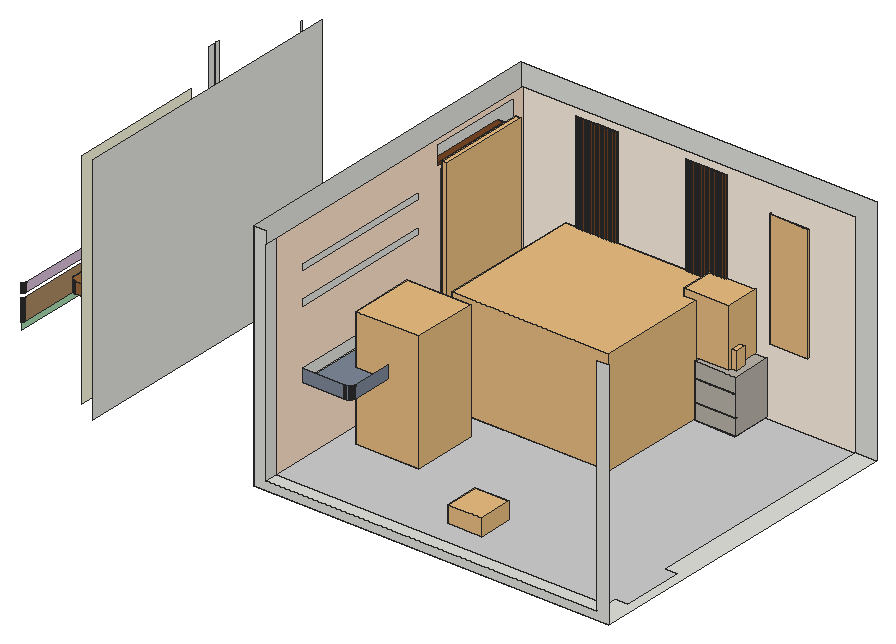
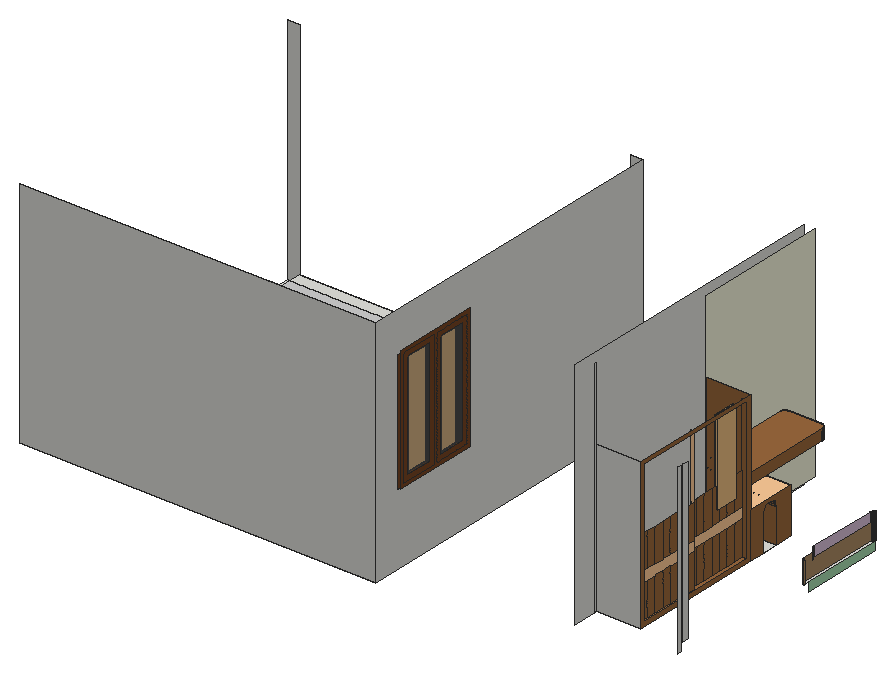
# SketchUp Ruby script. Lengths in inches.
U = 1.inch
M = Sketchup.active_model
def pt(a) = Geom::Point3d.new(a.map { |v| v * U })
def face(e, loops, mat)
  f = e.add_face(loops[0].map { |a| pt(a) })
  loops[1..].each { |l| e.add_face(l.map { |a| pt(a) }).erase! }
  f.material = f.back_material = mat if mat
  f
end
# faces: each face lists its corners as indices into pts; further lists are holes
def faces(e, pts, list, mat = nil) = list.each { |f| face(e, (f[0].is_a?(Array) ? f : [f]).map { |l| l.map { |i| pts[i] } }, mat) }
# xy, xz, yz: faces in a plane at the given z, y or x. An outline is a flat list of corners, or four numbers for a rectangle; further outlines are holes
def ring(l) = l.size == 4 ? [[l[0], l[1]], [l[2], l[1]], [l[2], l[3]], [l[0], l[3]]] : l.each_slice(2).to_a
def flat(e, list, mat, &to3) = list.each { |f| face(e, (f[0].is_a?(Array) ? f : [f]).map { |l| ring(l).map { |u, v| to3.(u, v) } }, mat) }
def xy(e, z, list, mat = nil) = flat(e, list, mat) { |x, y| [x, y, z] }
def xz(e, y, list, mat = nil) = flat(e, list, mat) { |x, z| [x, y, z] }
def yz(e, x, list, mat = nil) = flat(e, list, mat) { |y, z| [x, y, z] }
def lines(e, pts, list) = list.each { |a, b| e.add_line(pt(pts[a]), pt(pts[b])) }
# prism: a flat outline (further loops are holes) pulled along v
def prism(e, loops, v, mat = nil)
  f = face(e, loops, mat); d = Geom::Vector3d.new(v.map { |x| x * U })
  f.pushpull(f.normal.samedirection?(d) ? d.length : -d.length)
end
def box(e, o, s, mat = nil) = prism(e, [[o, [o[0] + s[0], o[1], o[2]], [o[0] + s[0], o[1] + s[1], o[2]], [o[0], o[1] + s[1], o[2]]]], [0, 0, s[2]], mat)
def at(x, y, z, deg = 0) = Geom::Transformation.translation(pt([x, y, z])) * Geom::Transformation.rotation(ORIGIN, Z_AXIS, deg.degrees)
def axes(o, x, y, z) = Geom::Transformation.new([*x, 0, *y, 0, *z, 0, *pt(o).to_a, 1])
def part(name) = M.definitions.add(name)
# library, detail: a bought-in or finely detailed component or shape, given as its bounding box
def library(name, o, s) = part(name).tap { |d| box(d.entities, o, s) }
def detail(e, o, s) = box(e.add_group.entities, o, s)
def put(e, d, t, mat = nil) = e.add_instance(d, t).tap { |i| i.material = mat if mat }
def group(e, t, mat = nil) = e.add_group.tap { |g| g.transformation = t; g.material = mat if mat }.entities
root = M.entities
M.materials.add("Leather K01 Brown 12cm").color = [167, 219, 175]
M.materials.add("Maquette Wood B01 12cm\#2").color = [172, 139, 100]
M.materials.add("Stone E 150cm").color = [186, 180, 170]
M.materials.add("[0049_Beige]").color = [245, 245, 220]
M.materials.add("[0090_LightCyan]").color = [224, 255, 255]
M.materials.add("[0110_LightSlateGray]").color = [127, 136, 153]
M.materials.add("[0110_LightSlateGray]1").color = [119, 136, 153]
M.materials.add("[0118_Thistle]").color = [216, 191, 216]
M.materials.add("[Carrera Marble]1").color = [207, 207, 207]
M.materials.add("[Color C01]").color = [255, 229, 204]
M.materials.add("[Color C02]").color = [255, 204, 153]
M.materials.add("[Color D01]").color = [255, 242, 228]
M.materials.add("[Translucent Glass Gray]").color = [132, 132, 132]
M.materials["[Translucent Glass Gray]"].alpha = 0.25
M.materials.add("[Wood Floor]").color = [155, 105, 61]
M.materials.add("[Wood Veneer 01]").color = [120, 70, 37]
c1 = library("Group\#3",[-0.5,-0.5,0],[2.0625,15.625,59.375])
c2 = part("Group\#33")
xy(c2.entities,0,[[0,0,19.69,1.18]],"[Wood Veneer 01]")
xy(c2.entities,2.76,[[2.76,0,16.93,1.18]],"[Wood Veneer 01]")
xy(c2.entities,60.24,[[2.76,0,16.93,1.18]],"[Wood Veneer 01]")
xy(c2.entities,62.99,[[0,0,19.69,1.18]],"[Wood Veneer 01]")
xz(c2.entities,0,[[2.76,2.76,16.93,60.24]],"[Translucent Glass Gray]")
xz(c2.entities,0,[[[0,0,19.69,62.99],[2.76,2.76,16.93,60.24]]],"[Wood Veneer 01]")
xz(c2.entities,1.18,[[[0,0,19.69,62.99],[2.76,2.76,16.93,60.24]]],"[Wood Veneer 01]")
yz(c2.entities,0,[[0,0,1.18,62.99]],"[Wood Veneer 01]")
yz(c2.entities,2.76,[[0,2.76,1.18,60.24]],"[Wood Veneer 01]")
yz(c2.entities,16.93,[[0,2.76,1.18,60.24]],"[Wood Veneer 01]")
yz(c2.entities,19.69,[[0,0,1.18,62.99]],"[Wood Veneer 01]")
c3 = part("pintu 2")
put(c3.entities,c2,at(-21.65,-1.97,1.97,-90))
g1 = group(c3.entities,at(-21.65,0,0,-90))
prism(g1,[[[0,0,66.93],[0,0,0],[45.28,0,0],[45.28,0,66.93]],[[43.31,0,1.97],[23.62,0,1.97],[23.62,0,64.96],[43.31,0,64.96]],[[21.65,0,64.96],[21.65,0,1.97],[1.97,0,1.97],[1.97,0,64.96]]],[0,5.91,0],"[Wood Veneer 01]")
put(c3.entities,c2,at(-21.65,-23.62,1.97,-90))
c4 = part("jendela")
put(c4.entities,c3,axes([-219.28,-83.75,50.21],[0.9198,0,0],[0,1.36117,0],[0,0,1.3104]))
c5 = library("Curtains\#1",[0,0,0],[121.73,8.19,117.22])
c6 = library("Chair 233 024",[-11.33,-15.06,-0.01],[22.66,30.64,41.53])
c7 = library("Bed 49-09",[-38.66,-44.09,0],[77.05,88.65,36.46])
c8 = library("Dome Light\#1",[-12,-12,0],[24,24,12])
c9 = library("Vase 004",[-7.23,-6.39,-0.02],[13.74,12.68,17.81])
c10 = library("Candle 296 009",[-1.31,-1.31,-0.01],[2.62,2.62,4.3])
c11 = library("Group\#8",[-0.5,-0.5,0],[27.375,1.5625,82.0625])
xy(root,0,[[314.72,0,566.72,236.75]])
xy(root,6.125,[[323.37,0,558.07,8.65],[467.82,201.17,495.07,228.1]])
xy(root,6.125,[[323.37,8.65,558.07,8.65,558.07,16.33,566.72,16.33,566.72,59.9,558.07,59.9,558.07,228.1,323.37,228.1]],"[Carrera Marble]1")
xy(root,7.125,[[467.07,200.35,467.82,228.1],[467.82,200.35,496.26,201.17],[495.07,201.17,496.26,228.1]])
xy(root,7.375,[[159.88,62.61,191.32,98.61]])
xy(root,10.06,[[159.88,101.5625,163.32,101.5625,163.32,147.01,161.57,147.01,161.57,192.875,159.88,192.875]],"[Wood Floor]")
xy(root,13.375,[[113.43,46.51,113.43,109,113.57,108.99,113.82,108.94,114.07,108.86,114.31,108.74,114.52,108.6,114.72,108.43,114.89,108.23,115.04,108.01,115.15,107.78,115.24,107.53,115.29,107.27,115.31,107.01,115.31,47.45,115.29,47.2,115.24,46.95,115.16,46.71,115.06,46.51],[113.43,109,113.43,109.01,113.31,109.01]])
xy(root,17.92,[[467.07,200.35,496.26,201.73]],"[0110_LightSlateGray]1")
xy(root,18.625,[[467.07,200.35,496.26,201.73]],"[0110_LightSlateGray]1")
xy(root,33.36,[[467.07,200.35,496.26,201.42]],"[0110_LightSlateGray]1")
xy(root,34.0625,[[467.07,200.35,496.26,201.42]],"[0110_LightSlateGray]1")
xy(root,44.375,[[467.07,200.35,496.26,228.1]],"Stone E 150cm")
xy(root,50.21,[[314.72,153.92,323.37,217.92]])
xy(root,54.08,[[360.9375,227.98,375.125,228.1],[439.0625,227.98,453.25,228.1]])
xy(root,54.08,[[376.0625,227.98,390.25,228.1],[453.8125,227.98,468,228.1]],"[0090_LightCyan]")
xy(root,54.9,[[323.37,31.6,323.37,123.51,353.74,123.51,354.39,123.47,355.03,123.36,355.65,123.17,356.24,122.92,356.78,122.6,357.28,122.22,357.71,121.79,358.07,121.31,358.36,120.79,358.57,120.25,358.7,119.68,358.74,119.11,358.74,36,358.7,35.43,358.57,34.86,358.36,34.32,358.07,33.8,357.71,33.33,357.28,32.89,356.78,32.51,356.24,32.19,355.65,31.9375,355.03,31.75,354.39,31.64,353.74,31.6]],"[0110_LightSlateGray]")
xy(root,54.9375,[[362.14,227.98,362.96,228.1]])
xy(root,54.9375,[[362.14,227.04,362.96,227.98],[364,227.04,364.83,228.1],[365.86,227.04,366.69,228.1],[367.73,227.04,368.55,228.1],[369.59,227.04,370.42,228.1],
  [371.46,227.04,372.28,228.1],[373.32,227.04,374.15,228.1],[377.14,227.04,377.96,228.1],[379,227.04,379.83,228.1],[380.86,227.04,381.69,228.1],
  [382.73,227.04,383.55,228.1],[384.59,227.04,385.42,228.1],[386.46,227.04,387.28,228.1],[388.32,227.04,389.15,228.1],[440.07,227.04,440.9,228.1],
  [441.9375,227.04,442.76,228.1],[443.8,227.04,444.63,228.1],[445.67,227.04,446.49,228.1],[447.53,227.04,448.36,228.1],[449.4,227.04,450.22,228.1],
  [451.26,227.04,452.09,228.1],[455.01,227.04,455.84,227.98],[456.88,227.04,457.71,228.1],[458.76,227.04,459.58,228.1],[460.63,227.04,461.45,228.1],
  [462.5,227.04,463.33,228.1],[464.375,227.04,465.2,228.1],[466.25,227.04,467.07,228.1],[455.01,227.98,455.84,228.1]],"[Wood Veneer 01]")
xy(root,55.6875,[[164.87,30.24,164.22,30.28,163.58,30.41,162.96,30.62,162.375,30.9,161.83,31.27,161.34,31.7,160.91,32.1875,160.55,32.73,160.26,33.3125,160.05,33.93,159.92,34.57,159.88,35.22,159.88,98.61,191.32,98.61,191.32,35.24,191.28,34.58,191.15,33.94,190.9375,33.32,190.65,32.74,190.29,32.19,189.86,31.7,189.36,31.27,188.82,30.91,188.23,30.62,187.61,30.41,186.97,30.28,186.32,30.24]],"[Wood Floor]")
xy(root,63.3125,[[164.87,30.24,186.32,30.24,186.97,30.28,187.61,30.41,188.23,30.62,188.82,30.91,189.36,31.27,189.86,31.7,190.29,32.19,190.65,32.74,190.9375,33.32,191.15,33.94,191.28,34.58,191.32,35.24,191.32,98.61,159.88,98.61,159.88,35.22,159.92,34.57,160.05,33.93,160.26,33.3125,160.55,32.73,160.91,32.1875,161.34,31.7,161.83,31.27,162.375,30.9,162.96,30.62,163.58,30.41,164.22,30.28]],"[Wood Floor]")
xy(root,150.4375,[[362.14,227.98,362.96,228.1]])
xy(root,150.4375,[[362.14,227.04,362.96,227.98],[364,227.04,364.83,228.1],[365.86,227.04,366.69,228.1],[367.73,227.04,368.55,228.1],[369.59,227.04,370.42,228.1],
  [371.46,227.04,372.28,228.1],[373.32,227.04,374.15,228.1],[377.14,227.04,377.96,228.1],[379,227.04,379.83,228.1],[380.86,227.04,381.69,228.1],
  [382.73,227.04,383.55,228.1],[384.59,227.04,385.42,228.1],[386.46,227.04,387.28,228.1],[388.32,227.04,389.15,228.1],[440.07,227.04,440.9,228.1],
  [441.9375,227.04,442.76,228.1],[443.8,227.04,444.63,228.1],[445.67,227.04,446.49,228.1],[447.53,227.04,448.36,228.1],[449.4,227.04,450.22,228.1],
  [451.26,227.04,452.09,228.1],[455.01,227.04,455.84,227.98],[456.88,227.04,457.71,228.1],[458.76,227.04,459.58,228.1],[460.63,227.04,461.45,228.1],
  [462.5,227.04,463.33,228.1],[464.375,227.04,465.2,228.1],[466.25,227.04,467.07,228.1],[455.01,227.98,455.84,228.1]],"[Wood Veneer 01]")
xy(root,150.83,[[360.9375,227.98,375.125,228.1],[376.0625,227.98,390.25,228.1],[439.0625,227.98,453.25,228.1],[453.8125,227.98,468,228.1]],"[0090_LightCyan]")
xz(root,0,[[314.72,0,566.72,0,566.72,164.75,558.07,164.75,558.07,6.125,323.37,6.125,323.37,164.75,314.72,164.75]])
xz(root,30.24,[[164.87,55.6875,186.32,63.3125]],"[Wood Floor]")
xz(root,31.6,[[323.37,54.9,353.74,63.71]],"[0110_LightSlateGray]")
xz(root,98.61,[[159.88,7.375,191.32,39.875],[159.88,55.6875,191.32,63.3125]])
xz(root,98.61,[[159.88,7.375,191.13,113.1875]],"[Wood Floor]")
xz(root,101.5625,[[159.88,10.06,163.32,110.51]],"[Wood Floor]")
xz(root,123.51,[[323.37,54.9,353.74,63.71]],"[0110_LightSlateGray]")
xz(root,147.01,[[161.57,10.06,163.32,110.51]],"[Color C02]")
xz(root,153.92,[[314.72,50.21,323.37,136.125]])
xz(root,192.875,[[159.88,10.06,161.57,110.51]],"[Wood Floor]")
xz(root,195.82,[[159.88,7.375,191.32,113.1875]])
xz(root,200.35,[[467.07,7.125,496.26,17.92],[467.07,18.625,496.26,33.36],[467.07,34.0625,496.26,44.375]],"Stone E 150cm")
xz(root,201.17,[[467.82,6.125,495.07,7.125]],"[0110_LightSlateGray]1")
xz(root,201.42,[[467.07,33.36,496.26,34.0625]],"[0110_LightSlateGray]1")
xz(root,201.73,[[467.07,17.92,496.26,18.625]],"[0110_LightSlateGray]1")
xz(root,217.92,[[314.72,50.21,323.37,136.125]])
xz(root,227.04,[[362.14,54.9375,362.96,150.4375],[364,54.9375,364.83,150.4375],[365.86,54.9375,366.69,150.4375],[367.73,54.9375,368.55,150.4375],[369.59,54.9375,370.42,150.4375],
  [371.46,54.9375,372.28,150.4375],[373.32,54.9375,374.15,150.4375],[377.14,54.9375,377.96,150.4375],[379,54.9375,379.83,150.4375],[380.86,54.9375,381.69,150.4375],
  [382.73,54.9375,383.55,150.4375],[384.59,54.9375,385.42,150.4375],[386.46,54.9375,387.28,150.4375],[388.32,54.9375,389.15,150.4375],[440.07,54.9375,440.9,150.4375],
  [441.9375,54.9375,442.76,150.4375],[443.8,54.9375,444.63,150.4375],[445.67,54.9375,446.49,150.4375],[447.53,54.9375,448.36,150.4375],[449.4,54.9375,450.22,150.4375],
  [451.26,54.9375,452.09,150.4375],[455.01,54.9375,455.84,150.4375],[456.88,54.9375,457.71,150.4375],[458.76,54.9375,459.58,150.4375],[460.63,54.9375,461.45,150.4375],
  [462.5,54.9375,463.33,150.4375],[464.375,54.9375,465.2,150.4375],[466.25,54.9375,467.07,150.4375]],"[Wood Veneer 01]")
xz(root,227.98,[[[360.9375,54.08,375.125,150.83],[362.14,54.9375,362.96,150.4375]],[[376.0625,54.08,390.25,150.83],[377.26,54.9375,378.09,150.4375]],[[439.0625,54.08,453.25,150.83],[440.26,54.9375,441.09,150.4375]],[[453.8125,54.08,468,150.83],[455.01,54.9375,455.84,150.4375]]],"[0090_LightCyan]")
xz(root,228.1,[[467.82,6.125,467.82,7.125,467.07,7.125,467.07,44.375,496.26,44.375,496.26,7.125,495.07,7.125,495.07,6.125],[[360.9375,54.08,375.125,150.83],[362.14,54.9375,362.96,150.4375]],[362.14,54.9375,362.96,150.4375]])
xz(root,228.1,[[323.37,6.125,558.07,155.75]],"[Color D01]")
xz(root,236.75,[[314.72,0,566.72,164.75]])
yz(root,112.06,[[52.76,28.5,101.76,35]],"[0118_Thistle]")
yz(root,113.43,[[46.51,7.375,105.14,13.375]],"Leather K01 Brown 12cm")
yz(root,115.31,[[47.45,13.375,107.01,28.5]],"Maquette Wood B01 12cm\#2")
yz(root,125.77,[[203.13,7.375,205.19,125.75],[197.07,13.0625,200.94,125.75]])
yz(root,159.88,[[[98.61,7.375,195.82,113.1875],[101.5625,10.06,192.875,110.51]],[35.22,55.6875,98.61,63.3125]],"[Wood Floor]")
yz(root,161.57,[[147.01,34.06,192.875,41.06]],"[Color C02]")
yz(root,161.57,[[147.01,10.06,153.82,34.06],[153.82,10.06,160.63,34.06],[160.63,10.06,167.44,34.06],[167.44,10.06,174.25,34.06],[174.25,10.06,181.0625,34.06],
  [181.0625,10.06,187.875,34.06],[187.875,10.06,192.875,34.06],[147.01,41.06,153.82,65.06],[153.82,41.06,160.63,65.06],[160.63,41.06,167.44,65.06],
  [167.44,41.06,174.25,65.06],[174.25,41.06,181.0625,65.06],[181.0625,41.06,187.875,65.06],[187.875,41.06,192.875,65.06]],"[Wood Floor]")
yz(root,163.32,[[101.5625,34.06,147.01,41.06]],"[Color C02]")
yz(root,163.32,[[101.5625,10.06,108.3,34.06],[108.3,10.06,115.04,34.06],[115.04,10.06,121.79,34.06],[121.79,10.06,128.53,34.06],[128.53,10.06,135.27,34.06],
  [135.27,10.06,142.01,34.06],[142.01,10.06,147.01,34.06],[101.5625,41.06,108.3,65.06],[108.3,41.06,108.3,65.06,109.82,65.06,109.82,57.32,110.31,55.66,111.16,54.15,112.35,52.88,113.79,51.93,115.04,51.47,115.04,41.06],[115.04,41.06,115.04,51.47,115.42,51.33,117.14,51.13,118.86,51.33,120.48,51.93,121.79,52.79,121.79,41.06],
  [121.79,41.06,121.79,52.79,121.93,52.88,123.11,54.15,123.96,55.66,124.45,57.32,124.45,65.06,128.53,65.06,128.53,41.06],[128.53,41.06,135.27,65.06],[135.27,41.06,142.01,65.06],[142.01,41.06,147.01,65.06]],"[Wood Floor]")
yz(root,191.13,[[2.25,7.375,98.61,164.75]],"[0049_Beige]")
yz(root,191.32,[[62.61,7.375,98.61,39.875],[195.82,7.375,197.07,164.75],[35.24,55.6875,98.61,63.3125]])
yz(root,198.9375,[[2.25,0,205.19,164.75]])
yz(root,314.72,[[[0,0,236.75,164.75],[153.92,50.21,217.92,136.125]]])
yz(root,323.37,[[0,6.125,8.65,155.75]])
yz(root,323.37,[[[8.65,6.125,228.1,155.75],[153.92,50.21,217.92,136.125],[152.04,138.75,219.6,152.6875],[31.6,54.9,123.51,63.71],[31.6,102.15,136.04,107.71],[31.6,124.78,136.04,129.78]]],"[Color C01]")
yz(root,358.74,[[36,54.9,119.11,63.71]],"[0110_LightSlateGray]")
yz(root,360.9375,[[227.98,54.08,228.1,150.83]])
yz(root,362.14,[[227.98,54.9375,228.1,150.4375]])
yz(root,362.14,[[227.04,54.9375,227.98,150.4375]],"[Wood Veneer 01]")
yz(root,362.96,[[227.98,54.9375,228.1,150.4375]])
yz(root,362.96,[[227.04,54.9375,227.98,150.4375]],"[Wood Veneer 01]")
yz(root,364,[[227.04,54.9375,228.1,150.4375]],"[Wood Veneer 01]")
yz(root,364.83,[[227.04,54.9375,228.1,150.4375]],"[Wood Veneer 01]")
yz(root,365.86,[[227.04,54.9375,228.1,150.4375]],"[Wood Veneer 01]")
yz(root,366.69,[[227.04,54.9375,228.1,150.4375]],"[Wood Veneer 01]")
yz(root,367.73,[[227.04,54.9375,228.1,150.4375]],"[Wood Veneer 01]")
yz(root,368.55,[[227.04,54.9375,228.1,150.4375]],"[Wood Veneer 01]")
yz(root,369.59,[[227.04,54.9375,228.1,150.4375]],"[Wood Veneer 01]")
yz(root,370.42,[[227.04,54.9375,228.1,150.4375]],"[Wood Veneer 01]")
yz(root,371.46,[[227.04,54.9375,228.1,150.4375]],"[Wood Veneer 01]")
yz(root,372.28,[[227.04,54.9375,228.1,150.4375]],"[Wood Veneer 01]")
yz(root,373.32,[[227.04,54.9375,228.1,150.4375]],"[Wood Veneer 01]")
yz(root,374.15,[[227.04,54.9375,228.1,150.4375]],"[Wood Veneer 01]")
yz(root,375.125,[[227.98,54.08,228.1,150.83]],"[0090_LightCyan]")
yz(root,376.0625,[[227.98,54.08,228.1,150.83]],"[0090_LightCyan]")
yz(root,377.14,[[227.04,54.9375,228.1,150.4375]],"[Wood Veneer 01]")
yz(root,377.96,[[227.04,54.9375,228.1,150.4375]],"[Wood Veneer 01]")
yz(root,379,[[227.04,54.9375,228.1,150.4375]],"[Wood Veneer 01]")
yz(root,379.83,[[227.04,54.9375,228.1,150.4375]],"[Wood Veneer 01]")
yz(root,380.86,[[227.04,54.9375,228.1,150.4375]],"[Wood Veneer 01]")
yz(root,381.69,[[227.04,54.9375,228.1,150.4375]],"[Wood Veneer 01]")
yz(root,382.73,[[227.04,54.9375,228.1,150.4375]],"[Wood Veneer 01]")
yz(root,383.55,[[227.04,54.9375,228.1,150.4375]],"[Wood Veneer 01]")
yz(root,384.59,[[227.04,54.9375,228.1,150.4375]],"[Wood Veneer 01]")
yz(root,385.42,[[227.04,54.9375,228.1,150.4375]],"[Wood Veneer 01]")
yz(root,386.46,[[227.04,54.9375,228.1,150.4375]],"[Wood Veneer 01]")
yz(root,387.28,[[227.04,54.9375,228.1,150.4375]],"[Wood Veneer 01]")
yz(root,388.32,[[227.04,54.9375,228.1,150.4375]],"[Wood Veneer 01]")
yz(root,389.15,[[227.04,54.9375,228.1,150.4375]],"[Wood Veneer 01]")
yz(root,390.25,[[227.98,54.08,228.1,150.83]],"[0090_LightCyan]")
yz(root,439.0625,[[227.98,54.08,228.1,150.83]],"[0090_LightCyan]")
yz(root,440.07,[[227.04,54.9375,228.1,150.4375]],"[Wood Veneer 01]")
yz(root,440.9,[[227.04,54.9375,228.1,150.4375]],"[Wood Veneer 01]")
yz(root,441.9375,[[227.04,54.9375,228.1,150.4375]],"[Wood Veneer 01]")
yz(root,442.76,[[227.04,54.9375,228.1,150.4375]],"[Wood Veneer 01]")
yz(root,443.8,[[227.04,54.9375,228.1,150.4375]],"[Wood Veneer 01]")
yz(root,444.63,[[227.04,54.9375,228.1,150.4375]],"[Wood Veneer 01]")
yz(root,445.67,[[227.04,54.9375,228.1,150.4375]],"[Wood Veneer 01]")
yz(root,446.49,[[227.04,54.9375,228.1,150.4375]],"[Wood Veneer 01]")
yz(root,447.53,[[227.04,54.9375,228.1,150.4375]],"[Wood Veneer 01]")
yz(root,448.36,[[227.04,54.9375,228.1,150.4375]],"[Wood Veneer 01]")
yz(root,449.4,[[227.04,54.9375,228.1,150.4375]],"[Wood Veneer 01]")
yz(root,450.22,[[227.04,54.9375,228.1,150.4375]],"[Wood Veneer 01]")
yz(root,451.26,[[227.04,54.9375,228.1,150.4375]],"[Wood Veneer 01]")
yz(root,452.09,[[227.04,54.9375,228.1,150.4375]],"[Wood Veneer 01]")
yz(root,453.25,[[227.98,54.08,228.1,150.83]],"[0090_LightCyan]")
yz(root,453.8125,[[227.98,54.08,228.1,150.83]],"[0090_LightCyan]")
yz(root,455.01,[[227.04,54.9375,227.98,150.4375],[227.98,54.9375,228.1,150.4375]],"[Wood Veneer 01]")
yz(root,455.84,[[227.04,54.9375,227.98,150.4375],[227.98,54.9375,228.1,150.4375]],"[Wood Veneer 01]")
yz(root,456.88,[[227.04,54.9375,228.1,150.4375]],"[Wood Veneer 01]")
yz(root,457.71,[[227.04,54.9375,228.1,150.4375]],"[Wood Veneer 01]")
yz(root,458.76,[[227.04,54.9375,228.1,150.4375]],"[Wood Veneer 01]")
yz(root,459.58,[[227.04,54.9375,228.1,150.4375]],"[Wood Veneer 01]")
yz(root,460.63,[[227.04,54.9375,228.1,150.4375]],"[Wood Veneer 01]")
yz(root,461.45,[[227.04,54.9375,228.1,150.4375]],"[Wood Veneer 01]")
yz(root,462.5,[[227.04,54.9375,228.1,150.4375]],"[Wood Veneer 01]")
yz(root,463.33,[[227.04,54.9375,228.1,150.4375]],"[Wood Veneer 01]")
yz(root,464.375,[[227.04,54.9375,228.1,150.4375]],"[Wood Veneer 01]")
yz(root,465.2,[[227.04,54.9375,228.1,150.4375]],"[Wood Veneer 01]")
yz(root,466.25,[[227.04,54.9375,228.1,150.4375]],"[Wood Veneer 01]")
yz(root,467.07,[[200.35,7.125,200.35,17.92,201.73,17.92,201.73,18.625,200.35,18.625,200.35,33.36,201.42,33.36,201.42,34.0625,200.35,34.0625,200.35,44.375,228.1,44.375,228.1,7.125]],"Stone E 150cm")
yz(root,467.07,[[227.04,54.9375,228.1,150.4375]],"[Wood Veneer 01]")
yz(root,467.82,[[201.17,6.125,228.1,7.125]],"[0110_LightSlateGray]1")
yz(root,468,[[227.98,54.08,228.1,150.83]],"[0090_LightCyan]")
yz(root,495.07,[[201.17,6.125,228.1,7.125]],"[0110_LightSlateGray]1")
yz(root,496.26,[[200.35,7.125,228.1,7.125,228.1,44.375,200.35,44.375,200.35,34.0625,201.42,34.0625,201.42,33.36,200.35,33.36,200.35,18.625,201.73,18.625,201.73,17.92,200.35,17.92]],"Stone E 150cm")
p = [[113.62,45.53,28.5],[113.37,45.51,28.5],[113.37,45.51,13.375],[113.62,45.53,13.375],[113.87,45.58,28.5],[113.87,45.58,13.375],
  [114.11,45.66,28.5],[114.11,45.66,13.375],[114.34,45.77,28.5],[114.34,45.77,13.375],[114.55,45.91,28.5],[114.55,45.91,13.375],
  [114.74,46.08,28.5],[114.74,46.08,13.375],[114.9,46.27,28.5],[114.9,46.27,13.375],[115.05,46.48,28.5],[115.05,46.48,13.375],
  [115.16,46.71,28.5],[115.06,46.51,13.375],[115.16,46.71,13.375],[115.24,46.95,28.5],[115.24,46.95,13.375],[115.29,47.2,28.5],
  [115.29,47.2,13.375],[115.31,47.45,28.5],[115.31,47.45,13.375],[115.29,107.27,28.5],[115.31,107.01,28.5],[115.31,107.01,13.375],
  [115.29,107.27,13.375],[115.24,107.53,28.5],[115.24,107.53,13.375],[115.15,107.78,28.5],[115.15,107.78,13.375],[115.04,108.01,28.5],
  [115.04,108.01,13.375],[114.89,108.23,28.5],[114.89,108.23,13.375],[114.72,108.43,28.5],[114.72,108.43,13.375],[114.52,108.6,28.5],
  [114.52,108.6,13.375],[114.31,108.74,28.5],[114.31,108.74,13.375],[114.07,108.86,28.5],[114.07,108.86,13.375],[113.57,108.99,28.5],
  [113.82,108.94,28.5],[113.82,108.94,13.375],[113.57,108.99,13.375],[113.31,109.01,28.5],[113.43,109,13.375],[113.31,109.01,13.375],
  [110.49,49.59,35],[110.06,49.3,35],[110.06,49.3,28.5],[110.49,49.59,28.5],[110.88,49.93,35],[110.88,49.93,28.5],
  [111.23,50.33,35],[111.23,50.33,28.5],[111.52,50.76,35],[111.52,50.76,28.5],[111.75,51.23,35],[111.75,51.23,28.5],
  [111.92,51.73,35],[111.92,51.73,28.5],[112.02,52.24,35],[112.02,52.24,28.5],[112.06,52.76,35],[112.06,52.76,28.5],
  [112.02,102.28,35],[112.06,101.76,35],[112.06,101.76,28.5],[112.02,102.28,28.5],[111.92,102.8,35],[111.92,102.8,28.5],
  [111.75,103.29,35],[111.75,103.29,28.5],[111.52,103.76,35],[111.52,103.76,28.5],[111.23,104.2,35],[111.23,104.2,28.5],
  [110.88,104.59,35],[110.88,104.59,28.5],[110.49,104.93,35],[110.49,104.93,28.5],[110.06,105.22,35],[110.06,105.22,28.5],
  [163.32,117.14,51.13],[163.32,115.42,51.33],[162.26,115.42,51.33],[162.26,117.14,51.13],[163.32,118.86,51.33],[162.26,118.86,51.33],
  [163.32,115.04,51.47],[162.26,115.04,51.47],[163.32,120.48,51.93],[162.26,120.48,51.93],[163.32,121.79,52.79],[162.26,121.79,52.79],
  [163.32,121.93,52.88],[162.26,121.93,52.88],[163.32,123.11,54.15],[162.26,123.11,54.15],[163.32,123.96,55.66],[162.26,123.96,55.66],
  [354.39,31.64,63.71],[353.74,31.6,63.71],[353.74,31.6,54.9],[354.39,31.64,54.9],[355.03,31.75,63.71],[355.03,31.75,54.9],
  [355.65,31.9375,63.71],[355.65,31.9375,54.9],[356.24,32.19,63.71],[356.24,32.19,54.9],[356.78,32.51,63.71],[356.78,32.51,54.9],
  [357.28,32.89,63.71],[357.28,32.89,54.9],[357.71,33.33,63.71],[357.71,33.33,54.9],[358.07,33.8,63.71],[358.07,33.8,54.9],
  [358.36,34.32,63.71],[358.36,34.32,54.9],[358.57,34.86,63.71],[358.57,34.86,54.9],[358.7,35.43,63.71],[358.7,35.43,54.9],
  [358.74,36,63.71],[358.74,36,54.9],[358.7,119.68,63.71],[358.74,119.11,63.71],[358.74,119.11,54.9],[358.7,119.68,54.9],
  [358.57,120.25,63.71],[358.57,120.25,54.9],[358.36,120.79,63.71],[358.36,120.79,54.9],[358.07,121.31,63.71],[358.07,121.31,54.9],
  [357.71,121.79,63.71],[357.71,121.79,54.9],[357.28,122.22,63.71],[357.28,122.22,54.9],[356.78,122.6,63.71],[356.78,122.6,54.9],
  [356.24,122.92,63.71],[356.24,122.92,54.9],[355.65,123.17,63.71],[355.65,123.17,54.9],[355.03,123.36,63.71],[355.03,123.36,54.9],
  [354.39,123.47,63.71],[354.39,123.47,54.9],[353.74,123.51,63.71],[353.74,123.51,54.9],[164.87,30.24,63.3125],[164.22,30.28,63.3125],
  [164.22,30.28,55.6875],[164.87,30.24,55.6875],[186.97,30.28,63.3125],[186.32,30.24,63.3125],[186.32,30.24,55.6875],[186.97,30.28,55.6875],
  [163.58,30.41,63.3125],[163.58,30.41,55.6875],[187.61,30.41,63.3125],[187.61,30.41,55.6875],[162.96,30.62,63.3125],[162.96,30.62,55.6875],
  [188.23,30.62,63.3125],[188.23,30.62,55.6875],[162.375,30.9,63.3125],[162.375,30.9,55.6875],[188.82,30.91,63.3125],[188.82,30.91,55.6875],
  [161.83,31.27,63.3125],[161.83,31.27,55.6875],[189.36,31.27,63.3125],[189.36,31.27,55.6875],[161.34,31.7,63.3125],[161.34,31.7,55.6875],
  [189.86,31.7,63.3125],[189.86,31.7,55.6875],[160.91,32.1875,63.3125],[160.91,32.1875,55.6875],[190.29,32.19,63.3125],[190.29,32.19,55.6875],
  [160.55,32.73,63.3125],[160.55,32.73,55.6875],[190.65,32.74,63.3125],[190.65,32.74,55.6875],[160.26,33.3125,63.3125],[160.26,33.3125,55.6875],
  [190.9375,33.32,63.3125],[190.9375,33.32,55.6875],[160.05,33.93,63.3125],[160.05,33.93,55.6875],[191.15,33.94,63.3125],[191.15,33.94,55.6875],
  [159.92,34.57,63.3125],[159.92,34.57,55.6875],[191.28,34.58,63.3125],[191.28,34.58,55.6875],[159.88,35.22,63.3125],[159.88,35.22,55.6875],
  [191.32,35.24,63.3125],[191.32,35.24,55.6875],[163.32,124.45,57.32],[162.26,124.45,57.32]]
faces(root,p,[[0,1,2,3],[4,0,3,5],[6,4,5,7],[8,6,7,9],[10,8,9,11],[12,10,11,13],[14,12,13,15],[16,14,15,17],
  [18,16,17,19,20],[21,18,20,22],[23,21,22,24],[25,23,24,26],[27,28,29,30],[31,27,30,32],[33,31,32,34],[35,33,34,36],
  [37,35,36,38],[39,37,38,40],[41,39,40,42],[43,41,42,44],[45,43,44,46],[47,48,49,50],[48,45,46,49],[51,47,50,52,53]],"Maquette Wood B01 12cm\#2")
faces(root,p,[[54,55,56,57],[58,54,57,59],[60,58,59,61],[62,60,61,63],[64,62,63,65],[66,64,65,67],[68,66,67,69],[70,68,69,71]],"[0118_Thistle]")
faces(root,p,[[72,73,74,75],[76,72,75,77],[78,76,77,79],[80,78,79,81],[82,80,81,83],[84,82,83,85],[86,84,85,87],[88,86,87,89],
  [90,91,92,93],[94,90,93,95],[91,96,97,92],[98,94,95,99],[100,98,99,101],[102,100,101,103],[104,102,103,105],[106,104,105,107],
  [212,106,107,213]])
faces(root,p,[[108,109,110,111],[112,108,111,113],[114,112,113,115],[116,114,115,117],[118,116,117,119],[120,118,119,121],[122,120,121,123],[124,122,123,125],
  [126,124,125,127],[128,126,127,129],[130,128,129,131],[132,130,131,133],[134,135,136,137],[138,134,137,139],[140,138,139,141],[142,140,141,143],
  [144,142,143,145],[146,144,145,147],[148,146,147,149],[150,148,149,151],[152,150,151,153],[154,152,153,155],[156,154,155,157],[158,156,157,159]],"[0110_LightSlateGray]")
faces(root,p,[[160,161,162,163],[164,165,166,167],[161,168,169,162],[170,164,167,171],[168,172,173,169],[174,170,171,175],[172,176,177,173],[178,174,175,179],
  [176,180,181,177],[182,178,179,183],[180,184,185,181],[186,182,183,187],[184,188,189,185],[190,186,187,191],[188,192,193,189],[194,190,191,195],
  [192,196,197,193],[198,194,195,199],[196,200,201,197],[202,198,199,203],[200,204,205,201],[206,202,203,207],[204,208,209,205],[210,206,207,211]],"[Wood Floor]")
put(root,c1,at(162.26,109.82,51.13))
g2 = group(root,at(159.88,62.61,7.375))
xy(g2,0,[[0,12.8125,14,24.9375]],"[Wood Floor]")
xy(g2,32.5,[[0,0,31.4375,36]],"[Color C02]")
xz(g2,0,[[0,0,31.4375,32.5]],"[Wood Floor]")
xz(g2,12.8125,[[0,0,14,24.33]],"[Wood Floor]")
xz(g2,24.9375,[[0,0,14,24.33]],"[Wood Floor]")
yz(g2,0,[[0,0,0,32.5,36,32.5,36,0,24.9375,0,24.9375,24.33,24.73,25.9,24.125,27.36,23.16,28.62,21.91,29.58,20.44,30.1875,18.875,30.39,17.31,30.1875,15.84,29.58,14.59,28.62,13.625,27.36,13.02,25.9,12.8125,24.33,12.8125,0]],"[Wood Floor]")
yz(g2,14,[[12.8125,0,12.8125,24.33,13.02,25.9,13.625,27.36,14.59,28.62,15.84,29.58,17.31,30.1875,18.875,30.39,20.44,30.1875,21.91,29.58,23.16,28.62,24.125,27.36,24.73,25.9,24.9375,24.33,24.9375,0]],"[Wood Floor]")
p = [[0,12.8125,24.33],[0,13.02,25.9],[14,13.02,25.9],[14,12.8125,24.33],[0,24.73,25.9],[0,24.9375,24.33],
  [14,24.9375,24.33],[14,24.73,25.9],[0,13.625,27.36],[14,13.625,27.36],[0,24.125,27.36],[14,24.125,27.36],
  [0,14.59,28.62],[14,14.59,28.62],[0,23.16,28.62],[14,23.16,28.62],[0,15.84,29.58],[14,15.84,29.58],
  [0,21.91,29.58],[14,21.91,29.58],[0,17.31,30.1875],[14,17.31,30.1875],[0,20.44,30.1875],[14,20.44,30.1875],
  [0,18.875,30.39],[14,18.875,30.39]]
faces(g2,p,[[0,1,2,3],[4,5,6,7],[1,8,9,2],[10,4,7,11],[8,12,13,9],[14,10,11,15],[12,16,17,13],[18,14,15,19],
  [16,20,21,17],[22,18,19,23],[20,24,25,21],[24,22,23,25]],"[Wood Floor]")
put(root,c4,at(553.54,299.29,0))
put(root,c5,axes([326.83,217.28,8.67],[0,-0.54,0],[0.41,0,0],[0,0,1.15]))
put(root,c6,axes([358.22,86.47,6.15],[0,-2.0207,0],[1.45842,0,0],[0,0,2.0207]))
put(root,c7,axes([409.57,177.125,6.125],[1.44305,0,0],[0,1.13212,0],[0,0,2.046]))
put(root,c8,at(444.4375,37.37,6.125))
put(root,c9,axes([472.97,218.875,44.4],[2.3,0,0],[0,2.3,0],[0,0,2.3]))
put(root,c10,axes([487.96,210.48,44.4],[2.76706,0,0],[0,2.9078,0],[0,0,2.9078]))
put(root,c11,at(499.2,227.54,54.9375))
